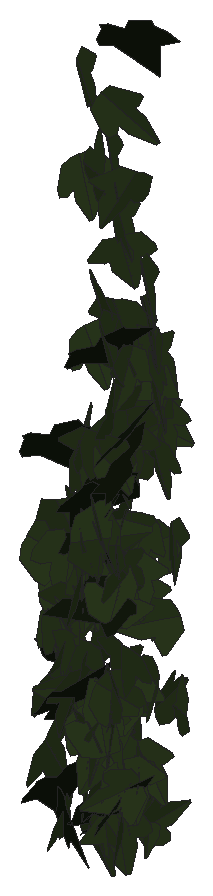
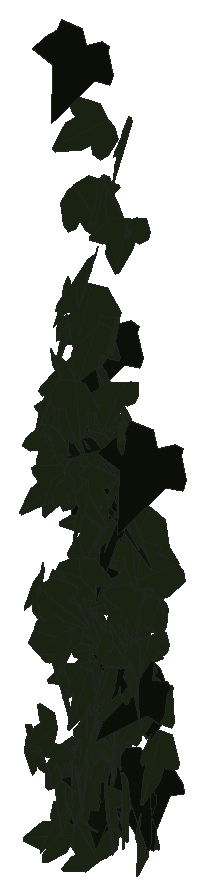
# SketchUp Ruby script. Lengths in inches.
U = 1.inch
M = Sketchup.active_model
def pt(a) = Geom::Point3d.new(a.map { |v| v * U })
def face(e, loops, mat)
  f = e.add_face(loops[0].map { |a| pt(a) })
  loops[1..].each { |l| e.add_face(l.map { |a| pt(a) }).erase! }
  f.material = f.back_material = mat if mat
  f
end
# faces: each face lists its corners as indices into pts; further lists are holes
def faces(e, pts, list, mat = nil) = list.each { |f| face(e, (f[0].is_a?(Array) ? f : [f]).map { |l| l.map { |i| pts[i] } }, mat) }
# xy, xz, yz: faces in a plane at the given z, y or x. An outline is a flat list of corners, or four numbers for a rectangle; further outlines are holes
def ring(l) = l.size == 4 ? [[l[0], l[1]], [l[2], l[1]], [l[2], l[3]], [l[0], l[3]]] : l.each_slice(2).to_a
def flat(e, list, mat, &to3) = list.each { |f| face(e, (f[0].is_a?(Array) ? f : [f]).map { |l| ring(l).map { |u, v| to3.(u, v) } }, mat) }
def xy(e, z, list, mat = nil) = flat(e, list, mat) { |x, y| [x, y, z] }
def xz(e, y, list, mat = nil) = flat(e, list, mat) { |x, z| [x, y, z] }
def yz(e, x, list, mat = nil) = flat(e, list, mat) { |y, z| [x, y, z] }
def lines(e, pts, list) = list.each { |a, b| e.add_line(pt(pts[a]), pt(pts[b])) }
# prism: a flat outline (further loops are holes) pulled along v
def prism(e, loops, v, mat = nil)
  f = face(e, loops, mat); d = Geom::Vector3d.new(v.map { |x| x * U })
  f.pushpull(f.normal.samedirection?(d) ? d.length : -d.length)
end
def box(e, o, s, mat = nil) = prism(e, [[o, [o[0] + s[0], o[1], o[2]], [o[0] + s[0], o[1] + s[1], o[2]], [o[0], o[1] + s[1], o[2]]]], [0, 0, s[2]], mat)
def at(x, y, z, deg = 0) = Geom::Transformation.translation(pt([x, y, z])) * Geom::Transformation.rotation(ORIGIN, Z_AXIS, deg.degrees)
def axes(o, x, y, z) = Geom::Transformation.new([*x, 0, *y, 0, *z, 0, *pt(o).to_a, 1])
def part(name) = M.definitions.add(name)
# library, detail: a bought-in or finely detailed component or shape, given as its bounding box
def library(name, o, s) = part(name).tap { |d| box(d.entities, o, s) }
def detail(e, o, s) = box(e.add_group.entities, o, s)
def put(e, d, t, mat = nil) = e.add_instance(d, t).tap { |i| i.material = mat if mat }
def group(e, t, mat = nil) = e.add_group.tap { |g| g.transformation = t; g.material = mat if mat }.entities
root = M.entities
M.materials.add("efeu1").color = [18, 25, 13]
M.materials.add("efeu2").color = [43, 57, 29]
c1 = part("ivyleaf_10")
p = [[0,0.5,-0.03],[-0.0625,2.02,-0.43],[-0.19,2.01,-0.46],[-0.54,1.05,-0.29],[-0.52,0.625,-0.18],[-0.83,0.76,-0.28],
  [-1.16,0.64,-0.33],[-1.15,0.33,-0.24],[-0.77,-0.39,0.02],[-0.3,-0.51,0.16],[0.04,-0.48,0.23],[-0.02,2.01,-0.4375],
  [-0.06,2.01,-0.43],[0.04,-0.49,0.23],[0.67,-0.49,0.14],[1.38,0.36,-0.2],[1.375,0.51,-0.24],[0.81,0.65,-0.19],
  [0.62,0.59,-0.15],[0.6,1.09,-0.28],[0.5,1.23,-0.31]]
faces(c1.entities,p,[[0,1,2,3,4,5,6,7,8,9,10],[11,12,0,13,14,15,16,17,18,19,20]],"efeu2")
c2 = part("ivyleaf_9")
p = [[1.54,2.16,1.25],[1.36,2.04,1.19],[-0.21,0.99,0.68],[-0.71,1.11,0.82],[-0.85,0.86,0.67],[-0.8,0.17,0.21],
  [-0.9,-0.01,0.1],[-0.67,-0.16,-0.02],[-0.08,-0.08,-0.05],[-0.03,-0.6,-0.4],[0.65,-0.88,-0.66],[0.83,-0.6,-0.49],
  [1.29,-0.42,-0.43],[1.8125,-0.07,-0.26],[1.21,0.44,0.15]]
faces(c2.entities,p,[[0,1,2,3,4,5,6,7,8,9,10,11,12,13,14]],"efeu1")
put(root,c1,axes([508.18,136.28,194.16],[-0.6792,-0.27391,0.11841],[-0.12185,-0.02597,-0.71305],[0.29629,-0.63858,-0.02179]))
put(root,c1,axes([508.45,136.125,197.3],[-0.32336,0.53903,0.14892],[-0.09295,0.11593,-0.64098],[-0.59513,-0.31098,0.01919]))
put(root,c1,axes([508.86,135.98,187.64],[-0.04929,0.05662,-0.63828],[-0.39597,0.49219,0.07558],[0.53506,0.36946,-0.00287]))
put(root,c1,axes([508.73,136.64,184.92],[0.17429,0.13276,-0.56771],[-0.4264,-0.37724,-0.21681],[-0.43163,0.42628,-0.01506]))
put(root,c2,axes([506.94,136.06,186.72],[0.22043,0.62544,-0.06793],[0.01628,0.06379,0.6842],[0.67896,-0.20458,0.00565]))
put(root,c1,axes([507.6,136.31,191.43],[-0.66864,0.24569,0.20045],[-0.26093,-0.10573,-0.66695],[-0.21366,-0.63974,0.1872]))
put(root,c1,axes([507.52,136.31,189.8],[-0.65327,-0.28582,0.08817],[-0.08896,-0.02407,-0.69563],[0.30945,-0.61032,-0.01386]))
put(root,c1,axes([506.74,136.09,185.64],[0.02106,-0.60352,-0.39627],[0.08135,0.3959,-0.59863],[0.71739,-0.02718,0.07951]))
put(root,c1,axes([507.23,136.54,187.34],[0.09079,-0.70124,0.16255],[0.03217,-0.15972,-0.707],[0.71911,0.09568,0.01111]))
put(root,c1,axes([507.22,136.32,191.03],[0.71857,0.22334,-0.06726],[-0.09889,0.0944,-0.74301],[-0.21125,0.71551,0.11902]))
put(root,c2,axes([506.64,136.57,183.89],[0.13589,-0.00723,-0.69321],[0.71828,-0.04434,0.13107],[-0.04851,-0.67687,-0.00118]))
put(root,c2,axes([508.97,136.28,194],[-0.5983,0.46887,0.06436],[-0.05665,0.03205,-0.76008],[-0.46987,-0.6009,0.00968]))
put(root,c2,axes([507.09,136.05,184.91],[0.11766,0.67631,-0.08721],[-0.01717,-0.08237,-0.71242],[-0.73581,0.11006,0.00268]))
put(root,c1,axes([508.07,135.86,191.76],[-0.05011,-0.0651,-0.78608],[0.54592,0.56567,-0.08165],[0.56933,-0.54814,0.0091]))
put(root,c1,axes([507.11,136.28,191.95],[-0.71872,-0.06482,-0.23032],[0.23251,-0.01725,-0.72073],[0.05643,-0.75453,0.03627]))
put(root,c1,axes([508.41,136.62,194.8],[-0.01816,-0.61705,-0.26897],[-0.01041,-0.25846,0.64196],[-0.7225,0.01923,-0.00249]))
put(root,c2,axes([508.17,136.32,192.91],[-0.02924,0.65607,-0.39234],[-0.01729,-0.3931,-0.65604],[-0.76424,-0.0162,0.02986]))
put(root,c1,axes([507.77,136,193.94],[0.21997,-0.21515,0.6127],[-0.39402,0.46319,0.3071],[-0.55097,-0.41715,0.02499]))
put(root,c1,axes([508.14,136.6875,185.98],[-0.48551,-0.39747,0.37014],[-0.11849,-0.40699,-0.59247],[0.53004,-0.45506,0.2066]))
put(root,c1,axes([507.58,136.27,186.51],[-0.58839,0.32277,0.07832],[-0.06966,0.03887,-0.65857],[-0.35111,-0.54861,-0.00059]))
put(root,c2,axes([508.53,136.57,190.1],[-0.63611,0.06245,0.30401],[-0.31722,-0.00097,-0.61526],[-0.05995,-0.65754,0.02978]))
put(root,c1,axes([507.46,136.41,193.28],[-0.08819,0.6241,-0.11878],[0.02055,-0.11269,-0.65458],[-0.68492,-0.08374,-0.00435]))
put(root,c1,axes([508.21,136.3,186.21],[0.27822,0.69295,-0.00425],[0.00154,0.00396,0.74672],[0.69296,-0.27823,0.00004]))
put(root,c1,axes([508.59,136.29,191.56],[-0.21651,0.14219,0.60156],[-0.63636,0.04209,-0.22314],[-0.09426,-0.61074,0.12468]))
put(root,c1,axes([506.81,136.5,189.85],[-0.67944,0.17274,-0.25591],[0.20463,-0.21125,-0.6859],[-0.2312,-0.69462,0.14496]))
put(root,c1,axes([507.53,136.26,190.25],[0.28312,-0.59272,-0.38248],[-0.06415,0.38879,-0.64999],[0.70249,0.27438,0.09479]))
put(root,c1,axes([507.34,136.47,188.34],[-0.57629,-0.14299,0.2352],[-0.22629,-0.09048,-0.57364],[0.17972,-0.57244,0.03191]))
put(root,c1,axes([507.74,136.41,191.95],[-0.18139,0.73538,-0.06968],[0.00674,-0.0701,-0.75735],[-0.73864,-0.18122,0.0102]))
put(root,c1,axes([508.79,136.39,188.68],[-0.67619,0.07405,0.15781],[-0.16588,-0.0077,-0.65517],[-0.07575,-0.64418,0.02597]))
put(root,c1,axes([508.78,136.21,184.32],[0.3188,-0.46577,-0.481],[-0.1304,0.47934,-0.5506],[0.65673,0.32127,0.12417]))
put(root,c1,axes([508.49,136.33,189.76],[0.53181,0.34404,-0.17014],[0.14255,0.09673,0.62472],[0.38595,-0.50979,0.00371]))
put(root,c1,axes([508,136.37,192.41],[-0.3683,0.66637,0.04571],[-0.04219,0.02889,-0.76103],[-0.66661,-0.37,0.02291]))
put(root,c2,axes([506.84,136.13,193.95],[0.49449,0.57643,-0.03673],[-0.01633,-0.03438,-0.7594],[-0.57737,0.49466,-0.00998]))
put(root,c1,axes([507.82,136.49,183.7],[-0.60266,0.21572,-0.1625],[0.15098,-0.07157,-0.62198],[-0.24487,-0.57505,0.01645]))
put(root,c1,axes([507.23,136.95,187],[-0.05621,-0.05586,-0.675],[-0.45741,-0.49181,0.07935],[-0.53457,0.42671,0.00309]))
put(root,c2,axes([508.26,136.04,196.91],[0.33376,0.69709,0.11537],[-0.01322,0.13373,-0.7698],[-0.70645,0.32684,0.06892]))
put(root,c1,axes([506.43,136.24,190.84],[0.24634,0.2079,0.65757],[0.4508,0.47593,-0.31935],[-0.5599,0.47466,0.03219]))
put(root,c2,axes([507.9,136.29,191.95],[-0.28955,0.56514,0.4192],[-0.31383,0.302,-0.6239],[-0.62978,-0.41032,0.11817]))
put(root,c1,axes([507.98,136.96,186.3125],[0.17329,-0.69293,0.32663],[0.09703,-0.31234,-0.71407],[0.75988,0.1979,0.0167]))
put(root,c2,axes([508.54,136.52,184.68],[-0.44333,0.54344,-0.04327],[0.02402,-0.03534,-0.70828],[-0.58814,-0.41108,0.00368]))
put(root,c1,axes([507.65,136.55,186.41],[0.56526,0.19179,0.44458],[0.40835,0.17836,-0.59614],[-0.26016,0.69667,0.03024]))
put(root,c1,axes([508.43,136.65,183.85],[-0.42686,-0.51943,-0.07955],[0.14444,-0.00702,-0.66911],[0.54833,-0.40251,0.11432]))
put(root,c1,axes([508.09,136.89,186.74],[0.41004,-0.44852,0.29566],[0.23646,-0.18618,-0.60957],[0.52249,0.43624,0.04383]))
put(root,c1,axes([507.54,136.75,190.23],[0.2381,0.57748,-0.19303],[-0.06972,-0.17403,-0.64286],[-0.65139,0.22971,-0.00175]))
put(root,c1,axes([508.64,136.84,196.32],[0.0661,0.51828,-0.3197],[-0.11751,-0.2944,-0.53874],[-0.6401,0.10756,0.06589]))
put(root,c1,axes([508.43,136.25,187.61],[0.22383,0.3349,0.53231],[0.07782,0.52329,-0.38643],[-0.656,0.17634,0.13578]))
put(root,c1,axes([506.91,136.64,189.82],[-0.4321,0.6065,-0.06494],[-0.00323,-0.08186,-0.74301],[-0.60996,-0.42922,0.04994]))
put(root,c2,axes([507.74,136.54,183.76],[0.42355,0.55705,-0.05595],[0.00797,0.06054,0.70788],[0.60436,-0.39119,0.02988]))
put(root,c1,axes([508.625,136.38,191.49],[-0.11138,0.26291,0.56905],[-0.4671,0.35763,-0.26349],[-0.46006,-0.42676,0.12976]))
put(root,c1,axes([506.7,136.42,187.28],[-0.21072,-0.48424,-0.52608],[0.21849,0.47861,-0.52806],[0.68082,-0.30348,0.00664]))
put(root,c1,axes([508.43,137.02,200.96],[-0.26119,-0.5212,0.31636],[-0.12788,-0.28036,-0.59748],[0.63909,-0.26911,0.00974]))
put(root,c2,axes([507.83,136.44,191.93],[0.43595,0.02046,-0.62236],[-0.60694,0.18376,-0.41912],[0.13917,0.7373,0.12172]))
put(root,c1,axes([508.25,136.625,193.96],[0.18075,0.56445,0.181],[0.05068,0.16762,-0.61228],[-0.63591,0.1738,0.00265]))
put(root,c1,axes([508.6,136.55,190.79],[-0.13076,-0.42922,-0.41438],[0.10957,0.38534,-0.46378],[0.62294,-0.15788,-0.00541]))
put(root,c1,axes([506.78,136.59,183.55],[0.06709,-0.44192,-0.39412],[-0.04414,0.37686,-0.46402],[0.62718,0.07379,0.0095]))
put(root,c1,axes([508.55,136.8125,194.75],[-0.40484,-0.46502,-0.04879],[0.03471,0.03434,-0.62117],[0.50357,-0.37621,0.0036]))
put(root,c2,axes([508.65,136.21,194.32],[0.18621,0.49207,0.5669],[-0.08409,0.59408,-0.48804],[-0.74595,0.05587,0.19653]))
put(root,c1,axes([508.57,136.72,185.22],[0.36827,0.50692,0.12701],[0.01245,0.13855,-0.6316],[-0.563,0.33465,0.06911]))
put(root,c1,axes([506.62,136.69,188.77],[0.0418,0.72857,0.11702],[-0.00644,0.11756,-0.72966],[-0.73788,0.04025,0.013]))
put(root,c1,axes([506.59,136.8,188.8],[0.21034,0.70534,0.0521],[0.02258,0.04763,-0.73599],[-0.7069,0.21139,-0.00801]))
put(root,c1,axes([506.76,136.73,189.92],[0.54884,0.3035,0.40505],[0.31573,0.2617,-0.62389],[-0.3956,0.62993,0.06403]))
put(root,c1,axes([507.2,136.73,191.69],[-0.48539,0.18763,0.38442],[-0.38285,0.10863,-0.50561],[-0.23206,-0.57168,0.03009]))
put(root,c1,axes([508.47,136.94,187.52],[0.47582,0.39182,-0.05045],[-0.03898,-0.03242,-0.61318],[-0.42461,0.44205,-0.00025]))
put(root,c1,axes([508.18,136.85,187.3125],[0.37983,-0.58871,-0.22389],[-0.05452,0.22974,-0.69658],[0.62748,0.37632,0.07501]))
put(root,c1,axes([506.78,136.9,188.2],[0.2075,-0.68416,-0.15987],[-0.02044,0.16075,-0.71445],[0.70229,0.20682,0.02645]))
put(root,c1,axes([508.11,136.77,203.01],[0.43167,0.00382,0.53812],[0.47523,0.34148,-0.35613],[-0.29402,0.55756,0.21443]))
put(root,c1,axes([507.78,136.75,201.06],[-0.07121,0.12682,0.67112],[-0.66189,0.2234,-0.11079],[-0.25763,-0.60898,0.09912]))
put(root,c1,axes([506.99,136.95,187.22],[0.16437,0.61063,0.01527],[0.00081,0.01495,-0.65448],[-0.65967,0.15217,0.003]))
put(root,c1,axes([507.22,136.86,184.625],[0.42796,-0.50023,-0.30869],[-0.05724,0.34456,-0.63771],[0.58501,0.39965,0.16343]))
put(root,c1,axes([507.84,137.47,191.4375],[-0.01175,-0.20861,-0.59787],[0.00186,-0.57497,0.21695],[-0.66047,0.00209,0.01125]))
put(root,c1,axes([508.32,136.9,196.3],[-0.29487,0.03603,0.57711],[-0.59593,0.05912,-0.28634],[-0.07449,-0.61561,0.00627]))
put(root,c1,axes([508.36,136.99,194.02],[-0.49473,-0.40592,-0.09271],[0.07202,0.05916,-0.63654],[0.44302,-0.46292,-0.00005]))
put(root,c2,axes([506.48,136.81,187.86],[0.7025,0.14553,-0.01792],[-0.0187,-0.00151,-0.6932],[-0.15716,0.65069,0.0024]))
put(root,c1,axes([507.49,137.02,197.72],[-0.49968,0.42792,-0.02321],[0.01979,-0.01305,-0.65542],[-0.46236,-0.46302,-0.00298]))
put(root,c1,axes([508.36,137.02,185.03],[-0.17569,-0.58924,-0.19265],[0.03942,0.18205,-0.6356],[0.66592,-0.16624,-0.0132]))
put(root,c2,axes([508.48,136.86,205.09],[0.5581,0.40239,-0.11224],[-0.07685,-0.08418,-0.68075],[-0.44333,0.52115,-0.02329]))
put(root,c2,axes([508.18,136.75,184.5],[-0.00452,0.63907,0.21841],[-0.08348,0.20816,-0.6604],[-0.7217,-0.02809,0.07503]))
put(root,c1,axes([508.26,137.25,185.05],[-0.57228,-0.34809,0.06832],[-0.02359,-0.08587,-0.65645],[0.38185,-0.527,0.06184]))
put(root,c1,axes([507.44,136.88,185.96],[0.20234,-0.32417,-0.56448],[-0.15885,0.52821,-0.3809],[0.66404,0.22514,0.08088]))
put(root,c1,axes([508.43,137.45,184.58],[-0.04621,-0.59832,0.21844],[0.05919,-0.21322,-0.62005],[0.68228,-0.02203,0.06859]))
put(root,c1,axes([508,137.16,197.33],[-0.64803,-0.09993,-0.09771],[0.09891,0.02195,-0.63259],[0.11027,-0.60694,-0.00679]))
put(root,c1,axes([507.45,136.91,188.23],[0.00274,-0.38539,-0.5406],[0.03747,0.51914,-0.40012],[0.69785,-0.02637,0.0236]))
put(root,c1,axes([508.42,137.2,190.43],[0.23284,0.54214,0.06855],[0.02571,0.06146,-0.60677],[-0.58927,0.2169,0.00061]))
put(root,c1,axes([507.33,137.29,184.56],[0.27803,-0.64417,-0.13141],[0.01266,0.1479,-0.6982],[0.65732,0.26962,0.06903]))
put(root,c1,axes([506.89,137.19,200.7],[0.30365,0.55016,0.10638],[0.00758,0.111,-0.64095],[-0.60431,0.27783,0.04542]))
put(root,c1,axes([506.95,137.15,203.36],[-0.32879,0.55973,0.13797],[-0.07953,0.11094,-0.66255],[-0.61614,-0.31301,0.01189]))
put(root,c1,axes([508.5,137.11,185.11],[0.3275,-0.3168,-0.50657],[-0.24416,0.44181,-0.44522],[0.57809,0.36607,0.09894]))
put(root,c1,axes([508.09,137.51,193.27],[-0.45434,-0.28942,0.34842],[-0.29218,-0.19776,-0.53099],[0.37848,-0.5001,0.00833]))
put(root,c1,axes([507.59,137.39,201.47],[-0.31462,0.55766,-0.08393],[0.00221,-0.0898,-0.65305],[-0.60854,-0.28864,0.04103]))
put(root,c1,axes([508.125,137.3,184.06],[-0.32118,0.52987,0.11871],[-0.10725,0.07472,-0.62985],[-0.57548,-0.30965,0.05113]))
put(root,c1,axes([507.02,137.31,196.1],[0.22336,0.55624,0.16725],[0.07596,0.14537,-0.61699],[-0.62071,0.21795,-0.01532]))
put(root,c1,axes([508.6,137.46,198.3125],[-0.31609,0.56041,-0.04001],[-0.01346,-0.04985,-0.65657],[-0.60652,-0.29096,0.03542]))
put(root,c1,axes([508.5,137.6,197.25],[-0.32232,0.49888,-0.2333],[0.11593,-0.19716,-0.60452],[-0.57926,-0.31704,0.00883]))
put(root,c1,axes([508.82,137.4,187.52],[0.33685,-0.38432,-0.41413],[-0.2582,0.31866,-0.51461],[0.53903,0.39281,0.0123]))
put(root,c1,axes([508.35,137.55,185.28],[0.49241,0.13067,0.36732],[0.35993,0.11826,-0.49293],[-0.18939,0.56448,0.01824]))
put(root,c1,axes([508,137.4,187.58],[-0.06175,-0.43754,-0.40817],[0.05573,0.38906,-0.45891],[0.63234,-0.07701,0.00059]))
put(root,c1,axes([508.55,137.72,196.46],[0.54957,-0.33325,-0.10419],[-0.06354,0.09254,-0.6309],[0.37042,0.5103,0.04636]))
put(root,c1,axes([508.8,137.94,188.9375],[0.17973,0.07715,-0.58842],[-0.56117,-0.22393,-0.19071],[-0.25575,0.54558,0.00493]))
put(root,c1,axes([507.71,137.69,198.69],[-0.45794,-0.42145,-0.13357],[0.13005,0.0606,-0.62029],[0.45772,-0.43888,0.04261]))
put(root,c1,axes([507.66,137.65,199.64],[-0.1854,0.59548,0.03929],[-0.00875,0.03698,-0.64452],[-0.64435,-0.17184,-0.00256]))
put(root,c1,axes([508,137.4,192.79],[-0.19443,0.34779,0.49026],[-0.28717,0.39092,-0.40555],[-0.56375,-0.31908,0.0375]))
put(root,c1,axes([507.71,137.62,186.48],[-0.43918,0.36673,0.15401],[-0.11255,0.10553,-0.56943],[-0.41205,-0.41971,-0.00861]))
put(root,c1,axes([507.85,137.71,184.72],[-0.5648,0.15905,0.10569],[-0.10328,0.03483,-0.56846],[-0.17575,-0.53161,-0.00562]))
put(root,c1,axes([508.37,137.97,183.71],[0.00935,0.49,-0.27716],[0.00228,-0.26656,-0.50965],[-0.60241,0.00659,-0.00623]))
put(root,c1,axes([508.61,137.84,195.29],[-0.22863,0.5561,-0.05625],[0.01121,-0.05391,-0.61875],[-0.60332,-0.21174,0.00982]))
put(root,c1,axes([506.68,138.17,189.81],[-0.04046,0.38406,-0.44789],[-0.06567,-0.43179,-0.39497],[-0.61973,0.02068,0.07109]))
put(root,c1,axes([506.5,138.09,189.34],[0.20678,-0.11964,-0.55329],[0.47735,-0.29617,0.2347],[-0.3449,-0.48164,-0.00689]))
put(root,c1,axes([508.51,137.875,194.46],[-0.59272,-0.222,-0.15796],[0.17482,0.00303,-0.61293],[0.23201,-0.56944,0.05832]))
put(root,c1,axes([508.58,137.9,193.46],[-0.58856,0.23574,-0.09552],[0.06294,-0.09528,-0.61397],[-0.26589,-0.54437,0.06609]))
put(root,c1,axes([508.32,137.99,195.29],[0.64021,-0.00773,0.07201],[0.0748,0.00123,-0.61655],[0.00814,0.59682,0.00221]))
put(root,c1,axes([507.76,137.71,185.97],[-0.41758,0.26792,0.32162],[-0.26951,0.18277,-0.48917],[-0.35019,-0.46014,-0.00704]))
put(root,c1,axes([507.49,137.65,183],[0.30536,0.46021,-0.31977],[0.18314,0.25664,0.56166],[0.56901,-0.32958,-0.00916]))
put(root,c1,axes([508.5,138.09,194.78],[0.56145,-0.25342,0.13744],[0.1327,-0.04951,-0.6014],[0.2787,0.53411,0.00947]))
put(root,c1,axes([508.22,137.625,185.28],[-0.12236,0.25681,-0.54597],[-0.20303,0.49031,0.29164],[0.59763,0.21915,-0.0127]))
put(root,c1,axes([507.96,138.23,193.79],[0.12602,0.4855,-0.32065],[-0.10102,-0.29439,-0.51893],[-0.61287,0.14836,0.0196]))
put(root,c1,axes([507.68,138.08,191.14],[-0.51495,-0.29208,0.06597],[-0.06531,-0.02268,-0.58139],[0.31612,-0.48047,-0.01265]))
put(root,c1,axes([508.67,137.77,195.97],[-0.19493,0.46476,0.35775],[-0.12733,0.32321,-0.51848],[-0.61135,-0.2155,-0.00608]))
put(root,c1,axes([507.8,138.12,196.14],[-0.62588,0.059,0.12167],[-0.13634,-0.10934,-0.593],[-0.0379,-0.58101,0.12396]))
put(root,c1,axes([508.43,137.8,183.28],[0.05513,-0.18085,0.57308],[0.00871,0.55333,0.18809],[-0.62629,-0.00822,0.05306]))
put(root,c1,axes([507.81,138.32,190.88],[0.59295,-0.04073,-0.09921],[-0.10137,0.02353,-0.57231],[0.04766,0.55676,0.01693]))
put(root,c1,axes([507.9,138.17,189.21],[0.05762,0.55438,0.0782],[0.01889,0.07384,-0.57912],[-0.60392,0.0552,-0.01066]))
put(root,c1,axes([508.13,138.64,190.55],[0.34619,0.03292,-0.47841],[-0.49807,0.02723,-0.33218],[0.00387,0.56002,0.04428]))
put(root,c1,axes([508.51,138.625,190.8],[-0.17998,0.52769,-0.10835],[-0.04316,-0.12092,-0.57045],[-0.5793,-0.15494,0.07617]))
put(root,c1,axes([508.47,138.27,186.4],[0.08587,-0.05345,0.57704],[-0.22446,0.5172,0.08279],[-0.55859,-0.21605,0.05543]))
put(root,c1,axes([508.01,138.43,193.69],[0.13688,0.29039,0.50109],[0.15209,0.4618,-0.32798],[-0.58822,0.18697,0.03181]))
put(root,c1,axes([508.76,138.65,186.13],[-0.0631,0.093,0.56631],[-0.56843,0.15693,-0.08661],[-0.18119,-0.52469,0.07447]))
